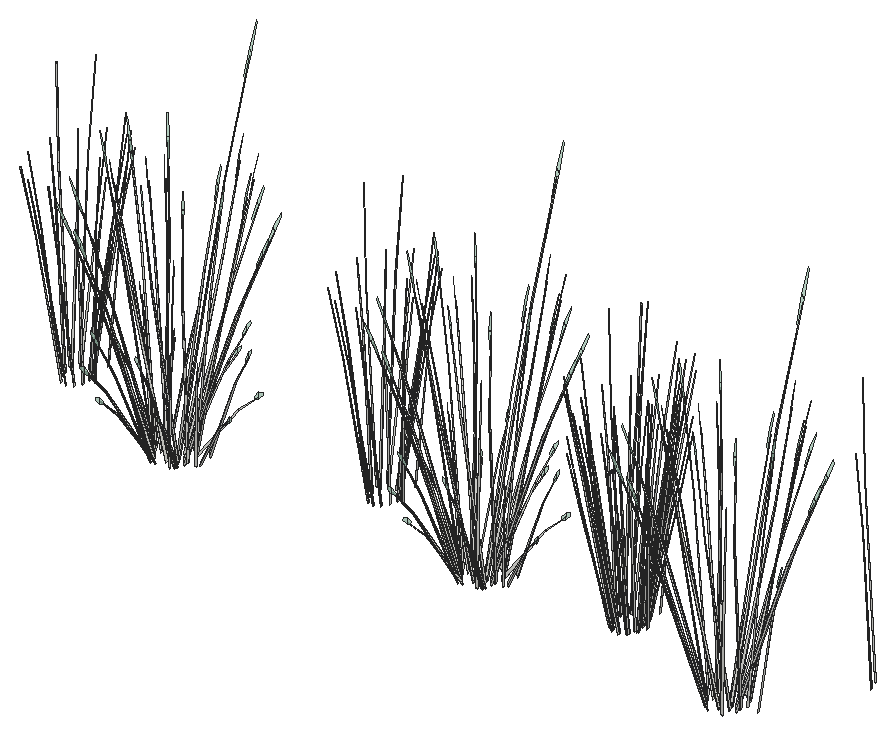
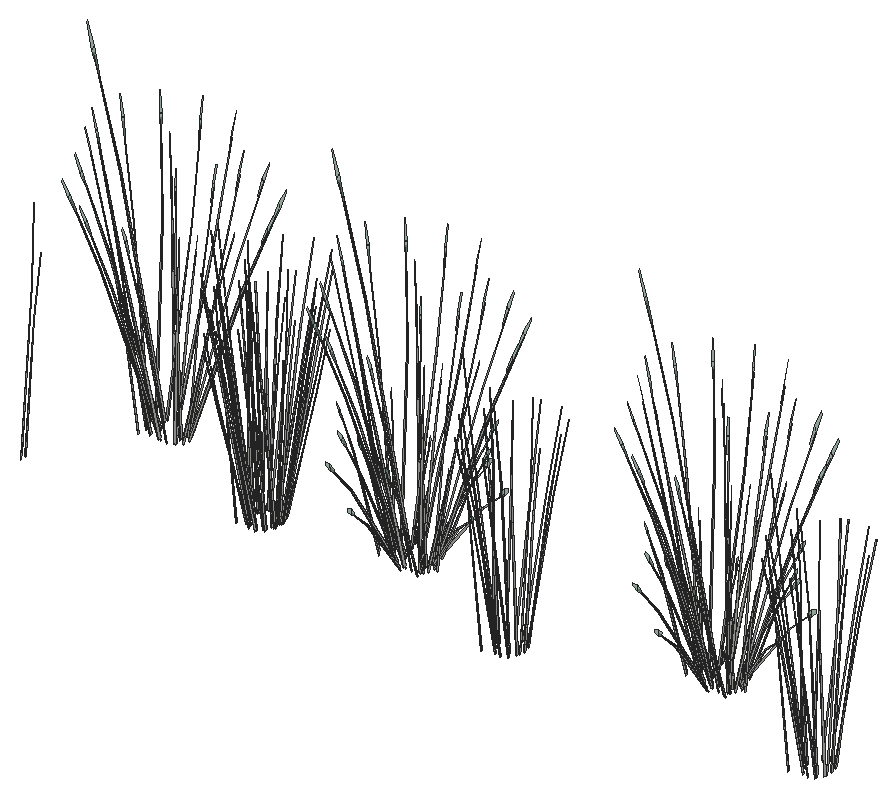
# SketchUp Ruby script. Lengths in inches.
U = 1.inch
M = Sketchup.active_model
def pt(a) = Geom::Point3d.new(a.map { |v| v * U })
def face(e, loops, mat)
  f = e.add_face(loops[0].map { |a| pt(a) })
  loops[1..].each { |l| e.add_face(l.map { |a| pt(a) }).erase! }
  f.material = f.back_material = mat if mat
  f
end
# faces: each face lists its corners as indices into pts; further lists are holes
def faces(e, pts, list, mat = nil) = list.each { |f| face(e, (f[0].is_a?(Array) ? f : [f]).map { |l| l.map { |i| pts[i] } }, mat) }
# xy, xz, yz: faces in a plane at the given z, y or x. An outline is a flat list of corners, or four numbers for a rectangle; further outlines are holes
def ring(l) = l.size == 4 ? [[l[0], l[1]], [l[2], l[1]], [l[2], l[3]], [l[0], l[3]]] : l.each_slice(2).to_a
def flat(e, list, mat, &to3) = list.each { |f| face(e, (f[0].is_a?(Array) ? f : [f]).map { |l| ring(l).map { |u, v| to3.(u, v) } }, mat) }
def xy(e, z, list, mat = nil) = flat(e, list, mat) { |x, y| [x, y, z] }
def xz(e, y, list, mat = nil) = flat(e, list, mat) { |x, z| [x, y, z] }
def yz(e, x, list, mat = nil) = flat(e, list, mat) { |y, z| [x, y, z] }
def lines(e, pts, list) = list.each { |a, b| e.add_line(pt(pts[a]), pt(pts[b])) }
# prism: a flat outline (further loops are holes) pulled along v
def prism(e, loops, v, mat = nil)
  f = face(e, loops, mat); d = Geom::Vector3d.new(v.map { |x| x * U })
  f.pushpull(f.normal.samedirection?(d) ? d.length : -d.length)
end
def box(e, o, s, mat = nil) = prism(e, [[o, [o[0] + s[0], o[1], o[2]], [o[0] + s[0], o[1] + s[1], o[2]], [o[0], o[1] + s[1], o[2]]]], [0, 0, s[2]], mat)
def at(x, y, z, deg = 0) = Geom::Transformation.translation(pt([x, y, z])) * Geom::Transformation.rotation(ORIGIN, Z_AXIS, deg.degrees)
def axes(o, x, y, z) = Geom::Transformation.new([*x, 0, *y, 0, *z, 0, *pt(o).to_a, 1])
def part(name) = M.definitions.add(name)
# library, detail: a bought-in or finely detailed component or shape, given as its bounding box
def library(name, o, s) = part(name).tap { |d| box(d.entities, o, s) }
def detail(e, o, s) = box(e.add_group.entities, o, s)
def put(e, d, t, mat = nil) = e.add_instance(d, t).tap { |i| i.material = mat if mat }
def group(e, t, mat = nil) = e.add_group.tap { |g| g.transformation = t; g.material = mat if mat }.entities
root = M.entities
M.materials.add("LightPink_Translucent").color = [175, 214, 192]
M.materials["LightPink_Translucent"].alpha = 0.75
c1 = part("blade")
p = [[2.15,0.21,22],[0,0.17,0],[0.09,0.45,0],[2.18,0.31,22],[2.29,0.31,22],[0.38,0.45,0],
  [2.48,0.24,33],[2.49,0.24,33],[2.48,0.22,33]]
faces(c1.entities,p,[[0,1,2,3],[4,5,2,3],[6,3,4,7],[8,0,3,6]])
c2 = part("blade with seeds\#1")
put(c2.entities,c1,at(0,0,0))
c3 = part("seeds")
p = [[0.3,-0.1,1.38],[-0.01,-0.03,1.59],[-0.01,-0.03,0.03],[0.14,-0.07,-0.07],[0.29,-0.03,3],[0.15,0.01,3.11]]
faces(c3.entities,p,[[0,1,2,3],[1,0,4,5]],"LightPink_Translucent")
c4 = part("blade with seeds")
put(c4.entities,c1,at(0,0,0))
put(c4.entities,c3,axes([2.4,0.25,30.99],[1.5799,-0.05474,1.17369],[-0.12525,1.92788,0.29478],[-0.07173,-0.02425,1.56792]))
put(root,c2,axes([371.35,244.1,140.9],[-0.09794,-0.55379,0.44104],[0.38419,-0.09611,0.36366],[-0.11323,0.13024,0.91263]))
put(root,c2,axes([371.67,242.85,140.86],[0.29303,0.14987,0.29052],[-0.08547,0.43725,-0.37506],[-0.11798,0.04009,0.71765]))
put(root,c2,axes([372,241.91,140.86],[0.20062,0.33637,0.29052],[-0.22908,0.31842,-0.37506],[-0.11639,-0.04845,0.71765]))
put(root,c2,axes([371.72,243.9,140.86],[0.30692,-0.07678,0.29052],[0.08104,0.43892,-0.37506],[-0.08795,0.11789,0.71765]))
put(root,c2,axes([371.92,245.22,140.9],[-0.28121,-0.41055,0.44104],[0.29863,-0.35407,0.36366],[-0.05187,0.19262,0.91263]))
put(root,c2,axes([372.62,241.33,140.86],[0.05446,0.43273,0.29052],[-0.31131,0.11427,-0.37506],[-0.08362,-0.12401,0.71765]))
put(root,c2,axes([372.13,244.78,140.86],[0.23857,-0.28286,0.29052],[0.22584,0.32298,-0.37506],[-0.03436,0.1641,0.71765]))
put(root,c2,axes([373.36,241.26,140.86],[-0.1063,0.41315,0.29052],[-0.31012,-0.1205,-0.37506],[-0.02844,-0.16634,0.71765]))
put(root,c2,axes([372.8,245.24,140.86],[0.1063,-0.41315,0.29052],[0.31012,0.1205,-0.37506],[0.02844,0.16634,0.71765]))
put(root,c2,axes([374.03,241.72,140.86],[-0.23857,0.28286,0.29052],[-0.22584,-0.32298,-0.37506],[0.03436,-0.1641,0.71765]))
put(root,c2,axes([373.54,245.17,140.86],[-0.05446,-0.43273,0.29052],[0.31131,-0.11427,-0.37506],[0.08362,0.12401,0.71765]))
put(root,c2,axes([374.43,246.16,141.35],[0.10171,-0.43869,-0.05322],[0.31305,0.13494,-0.24131],[0.04753,0.07175,0.79594]))
put(root,c2,axes([374.44,242.6,140.86],[-0.30692,0.07678,0.29052],[-0.08104,-0.43892,-0.37506],[0.08795,-0.11789,0.71765]))
put(root,c2,axes([374.16,244.59,140.86],[-0.20062,-0.33637,0.29052],[0.22908,-0.31842,-0.37506],[0.11639,0.04845,0.71765]))
put(root,c2,axes([374.49,243.65,140.86],[-0.29303,-0.14987,0.29052],[0.08547,-0.43725,-0.37506],[0.11798,-0.04009,0.71765]))
put(root,c2,axes([375.54,243.06,141.35],[-0.2186,-0.34354,-0.05322],[0.23941,-0.31478,-0.24131],[0.06784,-0.02216,0.79594]))
put(root,c2,axes([374.73,243.65,140.87],[-0.09962,0.48986,0.43711],[-0.3275,-0.16751,0.36041],[0.12879,-0.02944,0.90448]))
put(root,c4,axes([388.66,235.6875,140.7],[0.19824,-0.01009,1.55952],[-0.13151,0.43714,0.1261],[-0.28251,-0.02704,0.66668]))
put(root,c4,axes([388.74,236.46,140.7],[0.16583,-0.0942,1.55952],[0.13961,0.43527,0.1261],[-0.26034,0.09838,0.66668]))
put(root,c4,axes([388.23,236.3,141.46],[-0.07805,0.05782,1.59199],[0.00664,0.42244,-0.25177],[-0.1789,0.05494,0.12768]))
put(root,c4,axes([389.03,234.99,140.7],[0.17753,0.07673,1.55952],[-0.36739,0.32188,0.1261],[-0.22898,-0.14521,0.66668]))
put(root,c4,axes([387.36,236.73,141.46],[0.061,0.01194,1.61419],[0.18869,0.39348,-0.15253],[-0.12486,0.10328,0.28566]))
put(root,c4,axes([388.6,234.55,141.46],[0.03543,0.04444,1.61419],[-0.17081,0.3995,-0.15253],[-0.17299,0.00289,0.28566]))
put(root,c4,axes([389,234.28,141.46],[-0.10283,-0.00314,1.59199],[-0.32739,0.31434,-0.25177],[-0.17468,-0.06423,0.12768]))
put(root,c4,axes([388.73,235.9,141.75],[0.24047,0.40325,-0.11066],[-0.4268,0.19816,-0.6142],[-0.17986,0.0532,0.93327]))
put(root,c4,axes([389.27,235.0625,141.75],[-0.02559,0.45289,-0.11066],[-0.48454,-0.01238,-0.6142],[-0.18661,-0.03146,0.93327]))
put(root,c4,axes([389.35,236.75,140.7],[0.11937,-0.13683,1.55952],[0.30141,0.36934,0.1261],[-0.20674,0.1682,0.66668]))
put(root,c4,axes([389.26,237.09,140.7],[0.08899,-0.15307,1.55952],[0.37333,0.31677,0.1261],[-0.16841,0.19743,0.66668]))
put(root,c4,axes([388.24,237.88,141.46],[-0.01188,0.08813,1.59199],[0.33715,0.30658,-0.25177],[-0.08826,0.14498,0.12768]))
put(root,c4,axes([388.75,236.86,141.75],[0.44211,0.24556,-0.11066],[-0.2547,0.35561,-0.6142],[-0.12491,0.12361,0.93327]))
put(root,c4,axes([390.1,233.39,141.46],[-0.00892,0.05338,1.61419],[-0.43976,0.19372,-0.15253],[-0.12941,-0.09903,0.28566]))
put(root,c4,axes([389.76,234.54,140.7],[0.10925,0.14298,1.55952],[-0.50484,0.12037,0.1261],[-0.1141,-0.22447,0.66668]))
put(root,c4,axes([388.21,238.79,141.46],[0.05422,-0.02689,1.61419],[0.44816,0.17884,-0.15253],[-0.01053,0.14891,0.28566]))
put(root,c4,axes([390.6,233.59,141.46],[-0.0731,-0.06244,1.59199],[-0.48785,0.03959,-0.25177],[-0.07786,-0.14934,0.12768]))
put(root,c4,axes([391.34,234.56,141.75],[-0.4677,0.20734,-0.11066],[-0.22984,-0.36799,-0.6142],[-0.06171,-0.15507,0.93327]))
put(root,c4,axes([390.07,237.41,140.7],[-0.0117,-0.17092,1.55952],[0.50701,0.11339,0.1261],[-0.03136,0.24358,0.66668]))
put(root,c4,axes([390.18,238.97,141.46],[0.06058,0.07171,1.59199],[0.48891,0.02817,-0.25177],[0.04916,0.15815,0.12768]))
put(root,c4,axes([390.29,238.15,141.75],[0.4677,-0.20734,-0.11066],[0.22984,0.36799,-0.6142],[0.06171,0.15507,0.93327]))
put(root,c4,axes([392.68,234.04,141.46],[-0.04854,0.03402,1.61419],[-0.47555,-0.11476,-0.15253],[-0.01722,-0.14844,0.28566]))
put(root,c4,axes([392.31,235.02,141.75],[-0.52527,-0.02206,-0.11066],[0.01436,-0.41777,-0.6142],[0.03649,-0.1609,0.93327]))
put(root,c4,axes([390.96,237.34,140.7],[-0.10925,-0.14298,1.55952],[0.50484,-0.12037,0.1261],[0.1141,0.22447,0.66668]))
put(root,c4,axes([391.73,235.88,141.24],[-0.41299,-0.23139,1.25837],[0.43608,-0.36026,0.54295],[0.13325,0.21711,1.21634]))
put(root,c4,axes([391.03,238.45,141.46],[0.00141,-0.05392,1.61419],[0.40958,-0.23787,-0.15253],[0.14227,0.0849,0.28566]))
put(root,c4,axes([392.79,234.36,141.46],[-0.00461,-0.08863,1.59199],[-0.38966,-0.25616,-0.25177],[0.06024,-0.15528,0.12768]))
put(root,c4,axes([391.47,234.79,140.7],[-0.08899,0.15307,1.55952],[-0.37333,-0.31677,0.1261],[0.16841,-0.19743,0.66668]))
put(root,c4,axes([391.41,238.13,141.75],[0.2848,-0.38119,-0.11066],[0.41244,0.21961,-0.6142],[0.14337,0.10769,0.93327]))
put(root,c4,axes([392.88,235.84,141.75],[-0.44211,-0.24556,-0.11066],[0.2547,-0.35561,-0.6142],[0.12491,-0.12361,0.93327]))
put(root,c4,axes([391.69,236.89,140.7],[-0.17753,-0.07673,1.55952],[0.36739,-0.32188,0.1261],[0.22898,0.14521,0.66668]))
put(root,c4,axes([393.97,235.74,141.46],[-0.06243,-0.00338,1.61419],[-0.25923,-0.3624,-0.15253],[0.1041,-0.11916,0.28566]))
put(root,c4,axes([392.36,237.64,141.75],[0.02559,-0.45289,-0.11066],[0.48454,0.01238,-0.6142],[0.18661,0.03146,0.93327]))
put(root,c4,axes([392.9,236.8,141.75],[-0.24047,-0.40325,-0.11066],[0.4268,-0.19816,-0.6142],[0.17986,-0.0532,0.93327]))
put(root,c4,axes([392.78,237.37,141.46],[0.10253,-0.00753,1.59199],[0.28122,-0.34598,-0.25177],[0.18237,0.04567,0.12768]))
put(root,c4,axes([393.86,238,141.46],[-0.04322,-0.03899,1.61419],[0.09454,-0.41791,-0.15253],[0.17023,-0.0267,0.28566]))
put(root,c4,axes([392.07,236.19,140.7],[-0.19824,0.01009,1.55952],[0.13151,-0.43714,0.1261],[0.28251,0.02704,0.66668]))
put(root,c4,axes([394.2,236.17,141.46],[0.06632,-0.06783,1.59199],[-0.08489,-0.4161,-0.25177],[0.16641,-0.07889,0.12768]))
put(root,c2,axes([409.55,244.1,140.9],[-0.09794,-0.55379,0.44104],[0.38419,-0.09611,0.36366],[-0.11323,0.13024,0.91263]))
put(root,c2,axes([409.86,242.85,140.86],[0.29303,0.14987,0.29052],[-0.08547,0.43725,-0.37506],[-0.11798,0.04009,0.71765]))
put(root,c2,axes([410.19,241.91,140.86],[0.20062,0.33637,0.29052],[-0.22908,0.31842,-0.37506],[-0.11639,-0.04845,0.71765]))
put(root,c2,axes([409.91,243.9,140.86],[0.30692,-0.07678,0.29052],[0.08104,0.43892,-0.37506],[-0.08795,0.11789,0.71765]))
put(root,c2,axes([410.11,245.22,140.9],[-0.28121,-0.41055,0.44104],[0.29863,-0.35407,0.36366],[-0.05187,0.19262,0.91263]))
put(root,c2,axes([410.8125,241.33,140.86],[0.05446,0.43273,0.29052],[-0.31131,0.11427,-0.37506],[-0.08362,-0.12401,0.71765]))
put(root,c2,axes([410.32,244.78,140.86],[0.23857,-0.28286,0.29052],[0.22584,0.32298,-0.37506],[-0.03436,0.1641,0.71765]))
put(root,c2,axes([411.56,241.26,140.86],[-0.1063,0.41315,0.29052],[-0.31012,-0.1205,-0.37506],[-0.02844,-0.16634,0.71765]))
put(root,c2,axes([410.99,245.24,140.86],[0.1063,-0.41315,0.29052],[0.31012,0.1205,-0.37506],[0.02844,0.16634,0.71765]))
put(root,c2,axes([412.22,241.72,140.86],[-0.23857,0.28286,0.29052],[-0.22584,-0.32298,-0.37506],[0.03436,-0.1641,0.71765]))
put(root,c2,axes([411.74,245.17,140.86],[-0.05446,-0.43273,0.29052],[0.31131,-0.11427,-0.37506],[0.08362,0.12401,0.71765]))
put(root,c2,axes([412.62,246.16,141.35],[0.10171,-0.43869,-0.05322],[0.31305,0.13494,-0.24131],[0.04753,0.07175,0.79594]))
put(root,c2,axes([412.64,242.6,140.86],[-0.30692,0.07678,0.29052],[-0.08104,-0.43892,-0.37506],[0.08795,-0.11789,0.71765]))
put(root,c2,axes([412.36,244.59,140.86],[-0.20062,-0.33637,0.29052],[0.22908,-0.31842,-0.37506],[0.11639,0.04845,0.71765]))
put(root,c2,axes([412.6875,243.65,140.86],[-0.29303,-0.14987,0.29052],[0.08547,-0.43725,-0.37506],[0.11798,-0.04009,0.71765]))
put(root,c2,axes([413.73,243.06,141.35],[-0.2186,-0.34354,-0.05322],[0.23941,-0.31478,-0.24131],[0.06784,-0.02216,0.79594]))
put(root,c2,axes([412.93,243.65,140.87],[-0.09962,0.48986,0.43711],[-0.3275,-0.16751,0.36041],[0.12879,-0.02944,0.90448]))
put(root,c4,axes([426.85,235.6875,140.7],[0.19824,-0.01009,1.55952],[-0.13151,0.43714,0.1261],[-0.28251,-0.02704,0.66668]))
put(root,c4,axes([426.93,236.46,140.7],[0.16583,-0.0942,1.55952],[0.13961,0.43527,0.1261],[-0.26034,0.09838,0.66668]))
put(root,c4,axes([426.43,236.3,141.46],[-0.07805,0.05782,1.59199],[0.00664,0.42244,-0.25177],[-0.1789,0.05494,0.12768]))
put(root,c4,axes([427.23,234.99,140.7],[0.17753,0.07673,1.55952],[-0.36739,0.32188,0.1261],[-0.22898,-0.14521,0.66668]))
put(root,c4,axes([425.56,236.73,141.46],[0.061,0.01194,1.61419],[0.18869,0.39348,-0.15253],[-0.12486,0.10328,0.28566]))
put(root,c4,axes([426.8,234.55,141.46],[0.03543,0.04444,1.61419],[-0.17081,0.3995,-0.15253],[-0.17299,0.00289,0.28566]))
put(root,c4,axes([427.19,234.28,141.46],[-0.10283,-0.00314,1.59199],[-0.32739,0.31434,-0.25177],[-0.17468,-0.06423,0.12768]))
put(root,c4,axes([426.93,235.9,141.75],[0.24047,0.40325,-0.11066],[-0.4268,0.19816,-0.6142],[-0.17986,0.0532,0.93327]))
put(root,c4,axes([427.47,235.0625,141.75],[-0.02559,0.45289,-0.11066],[-0.48454,-0.01238,-0.6142],[-0.18661,-0.03146,0.93327]))
put(root,c4,axes([427.54,236.75,140.7],[0.11937,-0.13683,1.55952],[0.30141,0.36934,0.1261],[-0.20674,0.1682,0.66668]))
put(root,c4,axes([427.45,237.09,140.7],[0.08899,-0.15307,1.55952],[0.37333,0.31677,0.1261],[-0.16841,0.19743,0.66668]))
put(root,c4,axes([426.4375,237.88,141.46],[-0.01188,0.08813,1.59199],[0.33715,0.30658,-0.25177],[-0.08826,0.14498,0.12768]))
put(root,c4,axes([426.95,236.86,141.75],[0.44211,0.24556,-0.11066],[-0.2547,0.35561,-0.6142],[-0.12491,0.12361,0.93327]))
put(root,c4,axes([428.29,233.39,141.46],[-0.00892,0.05338,1.61419],[-0.43976,0.19372,-0.15253],[-0.12941,-0.09903,0.28566]))
put(root,c4,axes([427.96,234.54,140.7],[0.10925,0.14298,1.55952],[-0.50484,0.12037,0.1261],[-0.1141,-0.22447,0.66668]))
put(root,c4,axes([426.4,238.79,141.46],[0.05422,-0.02689,1.61419],[0.44816,0.17884,-0.15253],[-0.01053,0.14891,0.28566]))
put(root,c4,axes([428.79,233.59,141.46],[-0.0731,-0.06244,1.59199],[-0.48785,0.03959,-0.25177],[-0.07786,-0.14934,0.12768]))
put(root,c4,axes([429.53,234.56,141.75],[-0.4677,0.20734,-0.11066],[-0.22984,-0.36799,-0.6142],[-0.06171,-0.15507,0.93327]))
put(root,c4,axes([428.26,237.41,140.7],[-0.0117,-0.17092,1.55952],[0.50701,0.11339,0.1261],[-0.03136,0.24358,0.66668]))
put(root,c4,axes([428.38,238.97,141.46],[0.06058,0.07171,1.59199],[0.48891,0.02817,-0.25177],[0.04916,0.15815,0.12768]))
put(root,c4,axes([428.49,238.15,141.75],[0.4677,-0.20734,-0.11066],[0.22984,0.36799,-0.6142],[0.06171,0.15507,0.93327]))
put(root,c4,axes([430.88,234.04,141.46],[-0.04854,0.03402,1.61419],[-0.47555,-0.11476,-0.15253],[-0.01722,-0.14844,0.28566]))
put(root,c4,axes([430.5,235.02,141.75],[-0.52527,-0.02206,-0.11066],[0.01436,-0.41777,-0.6142],[0.03649,-0.1609,0.93327]))
put(root,c4,axes([429.16,237.34,140.7],[-0.10925,-0.14298,1.55952],[0.50484,-0.12037,0.1261],[0.1141,0.22447,0.66668]))
put(root,c4,axes([429.92,235.88,141.24],[-0.41299,-0.23139,1.25837],[0.43608,-0.36026,0.54295],[0.13325,0.21711,1.21634]))
put(root,c4,axes([429.23,238.45,141.46],[0.00141,-0.05392,1.61419],[0.40958,-0.23787,-0.15253],[0.14227,0.0849,0.28566]))
put(root,c4,axes([430.98,234.36,141.46],[-0.00461,-0.08863,1.59199],[-0.38966,-0.25616,-0.25177],[0.06024,-0.15528,0.12768]))
put(root,c4,axes([429.66,234.79,140.7],[-0.08899,0.15307,1.55952],[-0.37333,-0.31677,0.1261],[0.16841,-0.19743,0.66668]))
put(root,c4,axes([429.6,238.13,141.75],[0.2848,-0.38119,-0.11066],[0.41244,0.21961,-0.6142],[0.14337,0.10769,0.93327]))
put(root,c4,axes([431.08,235.84,141.75],[-0.44211,-0.24556,-0.11066],[0.2547,-0.35561,-0.6142],[0.12491,-0.12361,0.93327]))
put(root,c4,axes([429.89,236.89,140.7],[-0.17753,-0.07673,1.55952],[0.36739,-0.32188,0.1261],[0.22898,0.14521,0.66668]))
put(root,c4,axes([432.16,235.74,141.46],[-0.06243,-0.00338,1.61419],[-0.25923,-0.3624,-0.15253],[0.1041,-0.11916,0.28566]))
put(root,c4,axes([430.55,237.64,141.75],[0.02559,-0.45289,-0.11066],[0.48454,0.01238,-0.6142],[0.18661,0.03146,0.93327]))
put(root,c4,axes([431.09,236.8,141.75],[-0.24047,-0.40325,-0.11066],[0.4268,-0.19816,-0.6142],[0.17986,-0.0532,0.93327]))
put(root,c4,axes([430.97,237.37,141.46],[0.10253,-0.00753,1.59199],[0.28122,-0.34598,-0.25177],[0.18237,0.04567,0.12768]))
put(root,c4,axes([432.05,238,141.46],[-0.04322,-0.03899,1.61419],[0.09454,-0.41791,-0.15253],[0.17023,-0.0267,0.28566]))
put(root,c4,axes([430.26,236.19,140.7],[-0.19824,0.01009,1.55952],[0.13151,-0.43714,0.1261],[0.28251,0.02704,0.66668]))
put(root,c4,axes([432.4,236.17,141.46],[0.06632,-0.06783,1.59199],[-0.08489,-0.4161,-0.25177],[0.16641,-0.07889,0.12768]))
put(root,c2,axes([443.84,239.28,140.99],[-0.09794,-0.55379,0.44104],[0.38419,-0.09611,0.36366],[-0.11323,0.13024,0.91263]))
put(root,c2,axes([443.91,238.03,140.7],[0.09962,-0.48986,0.39379],[0.3275,0.16751,0.3247],[-0.12879,0.02944,0.81485]))
put(root,c2,axes([443.88,237.9,140.69],[-0.1295,-0.36632,0.05275],[0.23615,-0.1793,0.41527],[-0.1041,0.03538,0.63322]))
put(root,c2,axes([443.92,239.16,140.69],[-0.24206,-0.22594,0.05275],[0.14093,-0.32175,0.41527],[-0.07761,0.10402,0.63322]))
put(root,c2,axes([444.15,238.04,140.96],[0.29303,0.14987,0.29052],[-0.08547,0.43725,-0.37506],[-0.11798,0.04009,0.71765]))
put(root,c2,axes([443.89,239.05,141.27],[0.3653,0.33178,-0.11173],[-0.21045,0.48049,-0.62013],[-0.10321,0.16702,0.94228]))
put(root,c2,axes([444.27,236.92,140.7],[0.25999,-0.354,0.39379],[0.22422,0.37594,0.3247],[-0.12198,-0.0653,0.81485]))
put(root,c2,axes([444.3,236.79,140.69],[0.01775,-0.40853,0.05275],[0.2681,0.0112,0.41527],[-0.1027,-0.04275,0.63322]))
put(root,c2,axes([444.48,237.09,140.96],[0.20062,0.33637,0.29052],[-0.22908,0.31842,-0.37506],[-0.11639,-0.04845,0.71765]))
put(root,c2,axes([444.2,239.09,140.96],[0.30692,-0.07678,0.29052],[0.08104,0.43892,-0.37506],[-0.08795,0.11789,0.71765]))
put(root,c2,axes([444.4,240.4,140.99],[-0.28121,-0.41055,0.44104],[0.29863,-0.35407,0.36366],[-0.05187,0.19262,0.91263]))
put(root,c2,axes([444.4,240.22,140.69],[-0.28975,-0.02503,0.05275],[0.00794,-0.378,0.41527],[-0.03032,0.1448,0.63322]))
put(root,c2,axes([445.1,236.51,140.96],[0.05446,0.43273,0.29052],[-0.31131,0.11427,-0.37506],[-0.08362,-0.12401,0.71765]))
put(root,c2,axes([444.98,236.21,140.7],[0.35069,-0.12329,0.39379],[0.06086,0.48364,0.3247],[-0.08248,-0.14254,0.81485]))
put(root,c2,axes([445.05,236.12,140.69],[0.16025,-0.34128,0.05275],[0.22821,0.1987,0.41527],[-0.07378,-0.10942,0.63322]))
put(root,c2,axes([444.61,239.96,140.96],[0.23857,-0.28286,0.29052],[0.22584,0.32298,-0.37506],[-0.03436,0.1641,0.71765]))
put(root,c2,axes([445.84,236.44,140.96],[-0.1063,0.41315,0.29052],[-0.31012,-0.1205,-0.37506],[-0.02844,-0.16634,0.71765]))
put(root,c2,axes([445.28,240.76,140.7],[-0.34743,-0.14045,0.39379],[0.1188,-0.46175,0.3247],[0.02088,0.18159,0.81485]))
put(root,c2,axes([445.18,240.8,140.69],[-0.25981,0.18259,0.05275],[-0.12717,-0.33295,0.41527],[0.02509,0.14677,0.63322]))
put(root,c2,axes([445.94,236.07,140.69],[0.25981,-0.18259,0.05275],[0.12717,0.33295,0.41527],[-0.02509,-0.14677,0.63322]))
put(root,c2,axes([445.85,236.1,140.7],[0.34743,0.14045,0.39379],[-0.1188,0.46175,0.3247],[-0.02088,-0.18159,0.81485]))
put(root,c2,axes([445.28,240.43,140.96],[0.1063,-0.41315,0.29052],[0.31012,0.1205,-0.37506],[0.02844,0.16634,0.71765]))
put(root,c2,axes([446.51,236.9,140.96],[-0.23857,0.28286,0.29052],[-0.22584,-0.32298,-0.37506],[0.03436,-0.1641,0.71765]))
put(root,c2,axes([446.07,240.75,140.69],[-0.16025,0.34128,0.05275],[-0.22821,-0.1987,0.41527],[0.07378,0.10942,0.63322]))
put(root,c2,axes([446.14,240.65,140.7],[-0.35069,0.12329,0.39379],[-0.06086,-0.48364,0.3247],[0.08248,0.14254,0.81485]))
put(root,c2,axes([446.03,240.36,140.96],[-0.05446,-0.43273,0.29052],[0.31131,-0.11427,-0.37506],[0.08362,0.12401,0.71765]))
put(root,c2,axes([446.73,236.65,140.69],[0.28975,0.02503,0.05275],[-0.00794,0.378,0.41527],[0.03032,-0.1448,0.63322]))
put(root,c2,axes([446.64,236.61,140.7],[0.25108,0.36656,0.39379],[-0.26664,0.31614,0.3247],[0.04631,-0.17198,0.81485]))
put(root,c2,axes([446.91,241.34,141.44],[0.10171,-0.43869,-0.05322],[0.31305,0.13494,-0.24131],[0.04753,0.07175,0.79594]))
put(root,c2,axes([446.93,237.78,140.96],[-0.30692,0.07678,0.29052],[-0.08104,-0.43892,-0.37506],[0.08795,-0.11789,0.71765]))
put(root,c2,axes([446.65,239.77,140.96],[-0.20062,-0.33637,0.29052],[0.22908,-0.31842,-0.37506],[0.11639,0.04845,0.71765]))
put(root,c2,axes([446.83,240.08,140.69],[-0.01775,0.40853,0.05275],[-0.2681,-0.0112,0.41527],[0.1027,0.04275,0.63322]))
put(root,c2,axes([446.85,239.95,140.7],[-0.25999,0.354,0.39379],[-0.22422,-0.37594,0.3247],[0.12198,0.0653,0.81485]))
put(root,c2,axes([446.98,238.83,140.96],[-0.29303,-0.14987,0.29052],[0.08547,-0.43725,-0.37506],[0.11798,-0.04009,0.71765]))
put(root,c2,axes([447.21,237.71,140.69],[0.24206,0.22594,0.05275],[-0.14093,0.32175,0.41527],[0.07761,-0.10402,0.63322]))
put(root,c2,axes([447.14,237.61,140.7],[0.08745,0.49445,0.39379],[-0.34303,0.08581,0.3247],[0.1011,-0.11629,0.81485]))
put(root,c2,axes([448.02,238.24,141.44],[-0.2186,-0.34354,-0.05322],[0.23941,-0.31478,-0.24131],[0.06784,-0.02216,0.79594]))
put(root,c2,axes([447.24,238.96,140.69],[0.1295,0.36632,0.05275],[-0.23615,0.1793,0.41527],[0.1041,-0.03538,0.63322]))
put(root,c2,axes([446.7,239.99,141.24],[0.01888,-0.54637,-0.11073],[0.35746,0.01493,-0.6146],[0.13767,0.03795,0.93387]))
put(root,c2,axes([447.22,238.83,140.97],[-0.09962,0.48986,0.43711],[-0.3275,-0.16751,0.36041],[0.12879,-0.02944,0.90448]))
put(root,c4,axes([461.14,230.87,140.79],[0.19824,-0.01009,1.55952],[-0.13151,0.43714,0.1261],[-0.28251,-0.02704,0.66668]))
put(root,c4,axes([461.22,231.64,140.79],[0.16583,-0.0942,1.55952],[0.13961,0.43527,0.1261],[-0.26034,0.09838,0.66668]))
put(root,c4,axes([461.51,230.17,140.79],[0.17753,0.07673,1.55952],[-0.36739,0.32188,0.1261],[-0.22898,-0.14521,0.66668]))
put(root,c4,axes([461.21,231.08,141.85],[0.24047,0.40325,-0.11066],[-0.4268,0.19816,-0.6142],[-0.17986,0.0532,0.93327]))
put(root,c4,axes([461.75,230.25,141.85],[-0.02559,0.45289,-0.11066],[-0.48454,-0.01238,-0.6142],[-0.18661,-0.03146,0.93327]))
put(root,c4,axes([461.83,231.93,140.79],[0.11937,-0.13683,1.55952],[0.30141,0.36934,0.1261],[-0.20674,0.1682,0.66668]))
put(root,c4,axes([461.74,232.27,140.79],[0.08899,-0.15307,1.55952],[0.37333,0.31677,0.1261],[-0.16841,0.19743,0.66668]))
put(root,c4,axes([461.23,232.04,141.85],[0.44211,0.24556,-0.11066],[-0.2547,0.35561,-0.6142],[-0.12491,0.12361,0.93327]))
put(root,c4,axes([462.24,229.72,140.79],[0.10925,0.14298,1.55952],[-0.50484,0.12037,0.1261],[-0.1141,-0.22447,0.66668]))
put(root,c4,axes([463.82,229.74,141.85],[-0.4677,0.20734,-0.11066],[-0.22984,-0.36799,-0.6142],[-0.06171,-0.15507,0.93327]))
put(root,c4,axes([462.55,232.59,140.79],[-0.0117,-0.17092,1.55952],[0.50701,0.11339,0.1261],[-0.03136,0.24358,0.66668]))
put(root,c4,axes([462.78,233.33,141.85],[0.4677,-0.20734,-0.11066],[0.22984,0.36799,-0.6142],[0.06171,0.15507,0.93327]))
put(root,c4,axes([464.79,230.2,141.85],[-0.52527,-0.02206,-0.11066],[0.01436,-0.41777,-0.6142],[0.03649,-0.1609,0.93327]))
put(root,c4,axes([463.44,232.52,140.79],[-0.10925,-0.14298,1.55952],[0.50484,-0.12037,0.1261],[0.1141,0.22447,0.66668]))
put(root,c4,axes([464.21,231.07,141.34],[-0.41299,-0.23139,1.25837],[0.43608,-0.36026,0.54295],[0.13325,0.21711,1.21634]))
put(root,c4,axes([463.95,229.97,140.79],[-0.08899,0.15307,1.55952],[-0.37333,-0.31677,0.1261],[0.16841,-0.19743,0.66668]))
put(root,c4,axes([463.89,233.32,141.85],[0.2848,-0.38119,-0.11066],[0.41244,0.21961,-0.6142],[0.14337,0.10769,0.93327]))
put(root,c4,axes([465.36,231.03,141.85],[-0.44211,-0.24556,-0.11066],[0.2547,-0.35561,-0.6142],[0.12491,-0.12361,0.93327]))
put(root,c4,axes([465.96,232.83,140.84],[-0.09148,-0.37435,-0.03177],[0.43236,-0.08606,-0.14407],[0.09029,0.02373,0.47519]))
put(root,c4,axes([464.18,232.08,140.79],[-0.17753,-0.07673,1.55952],[0.36739,-0.32188,0.1261],[0.22898,0.14521,0.66668]))
put(root,c4,axes([464.84,232.82,141.85],[0.02559,-0.45289,-0.11066],[0.48454,0.01238,-0.6142],[0.18661,0.03146,0.93327]))
put(root,c4,axes([465.38,231.98,141.85],[-0.24047,-0.40325,-0.11066],[0.4268,-0.19816,-0.6142],[0.17986,-0.0532,0.93327]))
put(root,c4,axes([464.55,231.375,140.79],[-0.19824,0.01009,1.55952],[0.13151,-0.43714,0.1261],[0.28251,0.02704,0.66668]))
put(root,c2,axes([471.56,244.1,140.9],[-0.09794,-0.55379,0.44104],[0.38419,-0.09611,0.36366],[-0.11323,0.13024,0.91263]))
put(root,c2,axes([471.87,242.85,140.86],[0.29303,0.14987,0.29052],[-0.08547,0.43725,-0.37506],[-0.11798,0.04009,0.71765]))
